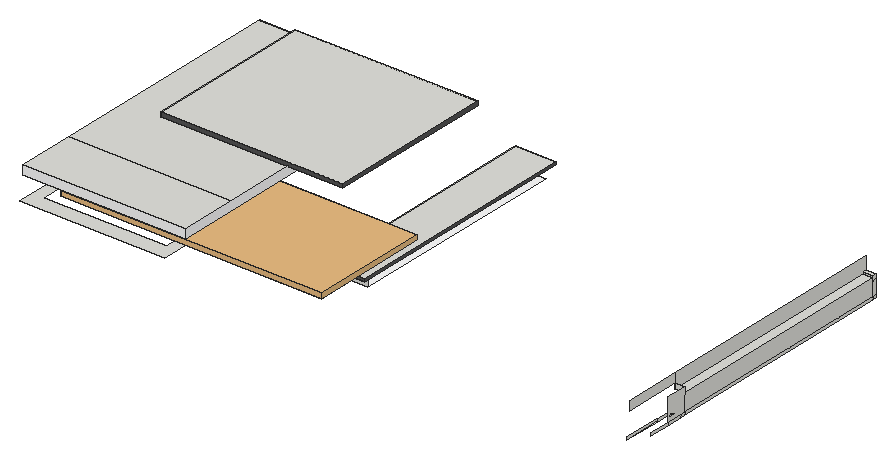
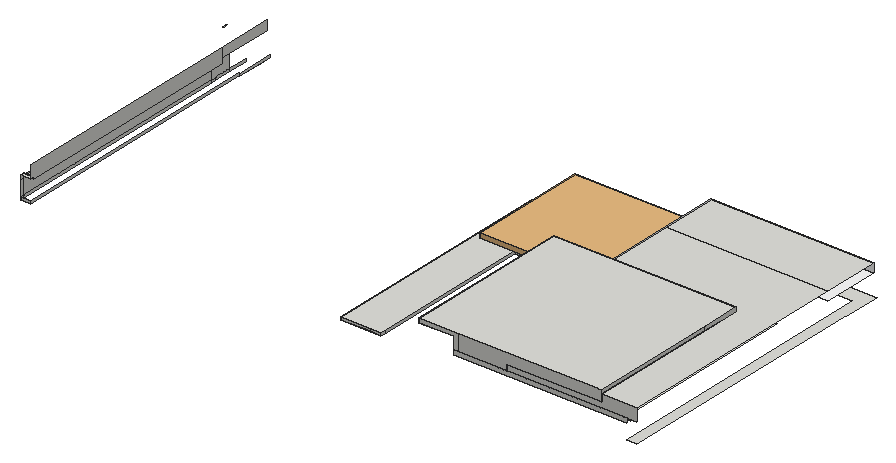
# SketchUp Ruby script. Lengths in inches.
U = 1.inch
M = Sketchup.active_model
def pt(a) = Geom::Point3d.new(a.map { |v| v * U })
def face(e, loops, mat)
  f = e.add_face(loops[0].map { |a| pt(a) })
  loops[1..].each { |l| e.add_face(l.map { |a| pt(a) }).erase! }
  f.material = f.back_material = mat if mat
  f
end
# faces: each face lists its corners as indices into pts; further lists are holes
def faces(e, pts, list, mat = nil) = list.each { |f| face(e, (f[0].is_a?(Array) ? f : [f]).map { |l| l.map { |i| pts[i] } }, mat) }
# xy, xz, yz: faces in a plane at the given z, y or x. An outline is a flat list of corners, or four numbers for a rectangle; further outlines are holes
def ring(l) = l.size == 4 ? [[l[0], l[1]], [l[2], l[1]], [l[2], l[3]], [l[0], l[3]]] : l.each_slice(2).to_a
def flat(e, list, mat, &to3) = list.each { |f| face(e, (f[0].is_a?(Array) ? f : [f]).map { |l| ring(l).map { |u, v| to3.(u, v) } }, mat) }
def xy(e, z, list, mat = nil) = flat(e, list, mat) { |x, y| [x, y, z] }
def xz(e, y, list, mat = nil) = flat(e, list, mat) { |x, z| [x, y, z] }
def yz(e, x, list, mat = nil) = flat(e, list, mat) { |y, z| [x, y, z] }
def lines(e, pts, list) = list.each { |a, b| e.add_line(pt(pts[a]), pt(pts[b])) }
# prism: a flat outline (further loops are holes) pulled along v
def prism(e, loops, v, mat = nil)
  f = face(e, loops, mat); d = Geom::Vector3d.new(v.map { |x| x * U })
  f.pushpull(f.normal.samedirection?(d) ? d.length : -d.length)
end
def box(e, o, s, mat = nil) = prism(e, [[o, [o[0] + s[0], o[1], o[2]], [o[0] + s[0], o[1] + s[1], o[2]], [o[0], o[1] + s[1], o[2]]]], [0, 0, s[2]], mat)
def at(x, y, z, deg = 0) = Geom::Transformation.translation(pt([x, y, z])) * Geom::Transformation.rotation(ORIGIN, Z_AXIS, deg.degrees)
def axes(o, x, y, z) = Geom::Transformation.new([*x, 0, *y, 0, *z, 0, *pt(o).to_a, 1])
def part(name) = M.definitions.add(name)
# library, detail: a bought-in or finely detailed component or shape, given as its bounding box
def library(name, o, s) = part(name).tap { |d| box(d.entities, o, s) }
def detail(e, o, s) = box(e.add_group.entities, o, s)
def put(e, d, t, mat = nil) = e.add_instance(d, t).tap { |i| i.material = mat if mat }
def group(e, t, mat = nil) = e.add_group.tap { |g| g.transformation = t; g.material = mat if mat }.entities
root = M.entities
M.materials.add("[Color M00]").color = [255, 255, 255]
M.materials.add("[Color M06]").color = [86, 86, 86]
c1 = library("Mesh Light\#4",[-0.5,-0.5,-0.1],[1,1,0.2])
c2 = part("Group\#24")
xy(c2.entities,0,[[203.13,95.41,201.58,95.62,200.13,96.22,198.89,97.17,197.9375,98.41,197.34,99.86,197.13,101.41,197.34,102.96,197.9375,104.41,198.89,105.65,200.13,106.61,201.58,107.21,203.13,107.41,204.6875,107.21,206.13,106.61,207.375,105.65,208.33,104.41,208.93,102.96,209.13,101.41,208.93,99.86,208.33,98.41,207.375,97.17,206.13,96.22,204.6875,95.62],[281.57,95.41,280.02,95.62,278.57,96.22,277.33,97.17,276.375,98.41,275.77,99.86,275.57,101.41,275.77,102.96,276.375,104.41,277.33,105.65,278.57,106.61,280.02,107.21,281.57,107.41,283.125,107.21,284.57,106.61,285.8125,105.65,286.77,104.41,287.37,102.96,287.57,101.41,287.37,99.86,286.77,98.41,285.8125,97.17,284.57,96.22,283.125,95.62],[350.95,95.41,349.39,95.62,347.95,96.22,346.7,97.17,345.75,98.41,345.15,99.86,344.95,101.41,345.15,102.96,345.75,104.41,346.7,105.65,347.95,106.61,349.39,107.21,350.95,107.41,352.5,107.21,353.95,106.61,355.1875,105.65,356.14,104.41,356.74,102.96,356.95,101.41,356.74,99.86,356.14,98.41,355.1875,97.17,353.95,96.22,352.5,95.62],[376,162.85,374.44,163.05,373,163.65,371.75,164.6,370.8,165.85,370.2,167.29,370,168.85,370.2,170.4,370.8,171.85,371.75,173.09,373,174.04,374.44,174.64,376,174.85,377.55,174.64,379,174.04,380.24,173.09,381.19,171.85,381.79,170.4,382,168.85,381.79,167.29,381.19,165.85,380.24,164.6,379,163.65,377.55,163.05]],"[Color M00]")
xy(c2.entities,33.4375,[[6,0,4.45,0.2,3,0.8,1.76,1.76,0.8,3,0.2,4.45,0,6,0.2,7.55,0.8,9,1.76,10.24,3,11.2,4.45,11.8,6,12,7.55,11.8,9,11.2,10.24,10.24,11.2,9,11.8,7.55,12,6,11.8,4.45,11.2,3,10.24,1.76,9,0.8,7.55,0.2],[83.125,0,81.57,0.2,80.125,0.8,78.88,1.76,77.93,3,77.33,4.45,77.125,6,77.33,7.55,77.93,9,78.88,10.24,80.125,11.2,81.57,11.8,83.125,12,84.68,11.8,86.125,11.2,87.37,10.24,88.32,9,88.92,7.55,89.125,6,88.92,4.45,88.32,3,87.37,1.76,86.125,0.8,84.68,0.2],[166.6875,0,165.13,0.2,163.6875,0.8,162.44,1.76,161.49,3,160.89,4.45,160.6875,6,160.89,7.55,161.49,9,162.44,10.24,163.6875,11.2,165.13,11.8,166.6875,12,168.24,11.8,169.6875,11.2,170.93,10.24,171.88,9,172.48,7.55,172.6875,6,172.48,4.45,171.88,3,170.93,1.76,169.6875,0.8,168.24,0.2],[166.6875,88.9375,165.13,89.14,163.6875,89.74,162.44,90.69,161.49,91.9375,160.89,93.38,160.6875,94.9375,160.89,96.49,161.49,97.9375,162.44,99.18,163.6875,100.13,165.13,100.73,166.6875,100.9375,168.24,100.73,169.6875,100.13,170.93,99.18,171.88,97.9375,172.48,96.49,172.6875,94.9375,172.48,93.38,171.88,91.9375,170.93,90.69,169.6875,89.74,168.24,89.14]],"[Color M00]")
put(c2.entities,c1,axes([191,87.42,16.72],[382.99758,0,0],[0,175.84579,0],[0,0,34.4375]))
c3 = library("Group\#23",[-0.5,-0.5,-0.1],[13,110.375,0.2])
xy(root,269.375,[[1170.95,1583.41,1383.39,1583.41,1383.39,1676.03,1376.89,1676.03,1376.89,1705.53,1367.875,1705.53,1367.875,1606.6875,1187.0625,1606.6875,1187.0625,2020.66,1172.33,2020.66,1172.33,1638.35,1170.95,1638.35],[1376.89,1676.03,1383.39,1730.6]])
xy(root,269.375,[[[1383.39,1676.03,1383.39,1730.6,1567.08,1730.6,1567.08,2001.02,1607.7,2001.02,1607.7,1676.03],[1418.61,1698.07,1420.16,1698.28,1421.61,1698.875,1422.85,1699.83,1423.8,1701.07,1424.4,1702.52,1424.61,1704.07,1424.4,1705.625,1423.8,1707.07,1422.85,1708.3125,1421.61,1709.27,1420.16,1709.87,1418.61,1710.07,1417.05,1709.87,1415.61,1709.27,1414.36,1708.3125,1413.41,1707.07,1412.81,1705.625,1412.61,1704.07,1412.81,1702.52,1413.41,1701.07,1414.36,1699.83,1415.61,1698.875,1417.05,1698.28],[1497.04,1698.07,1498.6,1698.28,1500.04,1698.875,1501.29,1699.83,1502.24,1701.07,1502.84,1702.52,1503.04,1704.07,1502.84,1705.625,1502.24,1707.07,1501.29,1708.3125,1500.04,1709.27,1498.6,1709.87,1497.04,1710.07,1495.49,1709.87,1494.04,1709.27,1492.8,1708.3125,1491.85,1707.07,1491.25,1705.625,1491.04,1704.07,1491.25,1702.52,1491.85,1701.07,1492.8,1699.83,1494.04,1698.875,1495.49,1698.28],[1566.42,1698.07,1567.97,1698.28,1569.42,1698.875,1570.66,1699.83,1571.61,1701.07,1572.21,1702.52,1572.42,1704.07,1572.21,1705.625,1571.61,1707.07,1570.66,1708.3125,1569.42,1709.27,1567.97,1709.87,1566.42,1710.07,1564.86,1709.87,1563.42,1709.27,1562.17,1708.3125,1561.22,1707.07,1560.62,1705.625,1560.42,1704.07,1560.62,1702.52,1561.22,1701.07,1562.17,1699.83,1563.42,1698.875,1564.86,1698.28],[1591.47,1765.51,1593.02,1765.71,1594.47,1766.31,1595.71,1767.26,1596.67,1768.51,1597.27,1769.95,1597.47,1771.51,1597.27,1773.06,1596.67,1774.51,1595.71,1775.75,1594.47,1776.7,1593.02,1777.3,1591.47,1777.51,1589.92,1777.3,1588.47,1776.7,1587.23,1775.75,1586.27,1774.51,1585.67,1773.06,1585.47,1771.51,1585.67,1769.95,1586.27,1768.51,1587.23,1767.26,1588.47,1766.31,1589.92,1765.71],[1591.47,1845.94,1593.02,1846.15,1594.47,1846.75,1595.71,1847.7,1596.67,1848.94,1597.27,1850.39,1597.47,1851.94,1597.27,1853.5,1596.67,1854.94,1595.71,1856.1875,1594.47,1857.14,1593.02,1857.74,1591.47,1857.94,1589.92,1857.74,1588.47,1857.14,1587.23,1856.1875,1586.27,1854.94,1585.67,1853.5,1585.47,1851.94,1585.67,1850.39,1586.27,1848.94,1587.23,1847.7,1588.47,1846.75,1589.92,1846.15],[1591.47,1943.32,1593.02,1943.52,1594.47,1944.12,1595.71,1945.08,1596.67,1946.32,1597.27,1947.77,1597.47,1949.32,1597.27,1950.87,1596.67,1952.32,1595.71,1953.5625,1594.47,1954.51,1593.02,1955.11,1591.47,1955.32,1589.92,1955.11,1588.47,1954.51,1587.23,1953.5625,1586.27,1952.32,1585.67,1950.87,1585.47,1949.32,1585.67,1947.77,1586.27,1946.32,1587.23,1945.08,1588.47,1944.12,1589.92,1943.52]]],"[Color M00]")
xy(root,270.375,[[2063.54,1592.1,2064.92,1636.04]])
xy(root,279.25,[[1376.89,1669.78,1607.7,1676.03],[1376.89,1676.03,1376.89,1775.97,1548.25,1775.97,1548.25,2020.66,1607.7,2020.66,1607.7,1676.03]])
xy(root,282.6875,[[1376.89,1669.78,1607.7,1669.78,1607.7,2020.66,1548.25,2020.66,1548.25,1775.97,1376.89,1775.97]])
xy(root,291.125,[[1197.375,1733.11,1197.375,2014.29,1364.27,2014.29,1364.27,1853.85,1354.74,1853.85,1354.74,1733.11],[1364.27,1853.85,1434.7,2014.29]])
xy(root,297.875,[[1187.0625,2014.29,1364.27,2020.66],[1364.27,2014.29,1434.7,2020.66]])
xy(root,299.625,[[2064.92,1667.53,2079.65,2011.98]])
xy(root,302.5625,[[2064.92,2011.98,2079.65,2018.36]])
xy(root,302.8125,[[[1172.33,1586.53,1172.33,1669.84,1187.0625,1669.84,1187.0625,1638.53,1364.27,1638.53,1364.27,1831.47,1410.7,1831.47,1410.7,1586.53],[1382.16,1691.6,1383.71,1691.8,1385.16,1692.4,1386.4,1693.35,1387.36,1694.6,1387.96,1696.04,1388.16,1697.6,1387.96,1699.15,1387.36,1700.6,1386.4,1701.84,1385.16,1702.79,1383.71,1703.39,1382.16,1703.6,1380.61,1703.39,1379.16,1702.79,1377.92,1701.84,1376.96,1700.6,1376.36,1699.15,1376.16,1697.6,1376.36,1696.04,1376.96,1694.6,1377.92,1693.35,1379.16,1692.4,1380.61,1691.8],[1221.47,1602.66,1223.03,1602.86,1224.47,1603.46,1225.71,1604.42,1226.67,1605.66,1227.27,1607.11,1227.47,1608.66,1227.27,1610.21,1226.67,1611.66,1225.71,1612.9,1224.47,1613.86,1223.03,1614.46,1221.47,1614.66,1219.92,1614.46,1218.47,1613.86,1217.23,1612.9,1216.28,1611.66,1215.68,1610.21,1215.47,1608.66,1215.68,1607.11,1216.28,1605.66,1217.23,1604.42,1218.47,1603.46,1219.92,1602.86],[1298.6,1602.66,1300.15,1602.86,1301.6,1603.46,1302.84,1604.42,1303.79,1605.66,1304.39,1607.11,1304.6,1608.66,1304.39,1610.21,1303.79,1611.66,1302.84,1612.9,1301.6,1613.86,1300.15,1614.46,1298.6,1614.66,1297.04,1614.46,1295.6,1613.86,1294.35,1612.9,1293.4,1611.66,1292.8,1610.21,1292.6,1608.66,1292.8,1607.11,1293.4,1605.66,1294.35,1604.42,1295.6,1603.46,1297.04,1602.86],[1382.16,1602.66,1383.71,1602.86,1385.16,1603.46,1386.4,1604.42,1387.36,1605.66,1387.96,1607.11,1388.16,1608.66,1387.96,1610.21,1387.36,1611.66,1386.4,1612.9,1385.16,1613.86,1383.71,1614.46,1382.16,1614.66,1380.61,1614.46,1379.16,1613.86,1377.92,1612.9,1376.96,1611.66,1376.36,1610.21,1376.16,1608.66,1376.36,1607.11,1376.96,1605.66,1377.92,1604.42,1379.16,1603.46,1380.61,1602.86]]],"[Color M00]")
xy(root,305.625,[[1224.7,1831.47,1364.27,2020.66]])
xy(root,316.0625,[[1172.33,1586.53,1410.7,1669.84],[1172.33,1669.84,1410.7,1669.84,1410.7,1773.85,1224.7,1773.85,1224.7,2020.66,1172.33,2020.66],[1410.7,1773.85,1410.7,1831.47,1440.7,1831.47,1440.7,2020.66,1492.27,2020.66,1492.27,1773.85]])
xy(root,321.8125,[[1224.7,1773.85,1492.27,2020.66]])
xz(root,1586.53,[[1172.33,302.8125,1410.7,316.0625]],"[Color M00]")
xz(root,1636.04,[[2063.54,270.375,2064.92,274.0625]])
xz(root,1667.53,[[2064.92,299.625,2079.65,307.5]])
xz(root,1669.78,[[1376.89,279.25,1607.7,282.6875]],"[Color M06]")
xz(root,1676.03,[[1376.89,269.375,1607.7,279.25]])
xz(root,1773.85,[[1224.7,316.0625,1492.27,321.8125]],"[Color M06]")
xz(root,1775.97,[[1376.89,279.25,1548.25,282.6875]])
xz(root,1831.47,[[1364.27,302.8125,1410.7,305.625]])
xz(root,2011.98,[[2064.92,299.625,2079.65,302.5625]])
xz(root,2014.29,[[1187.0625,291.125,1364.27,297.875],[1364.27,291.125,1434.7,297.875]])
xz(root,2018.36,[[2064.92,270.375,2079.65,274.0625]])
xz(root,2020.66,[[1548.25,279.25,1563.95,282.6875],[1563.95,279.25,1607.7,282.6875],[1187.0625,291.125,1440.7,297.875],[1172.33,297.875,1172.33,316.0625,1224.7,316.0625,1224.7,305.625,1364.27,305.625,1364.27,297.875],[1364.27,297.875,1364.27,305.625,1224.7,305.625,1224.7,321.8125,1434.7,321.8125,1434.7,297.875],
  [1434.7,297.875,1434.7,321.8125,1492.27,321.8125,1492.27,316.0625,1440.7,316.0625,1440.7,297.875]])
yz(root,1224.7,[[1803.47,305.625,1831.47,316.0625],[1831.47,305.625,2020.66,316.0625],[1773.85,316.0625,1831.47,321.8125],[1831.47,316.0625,2020.66,321.8125]])
yz(root,1364.27,[[1831.47,291.125,2014.29,297.875],[1831.47,297.875,2020.66,305.625]])
yz(root,1376.89,[[1669.78,279.25,1775.97,282.6875]])
yz(root,1410.7,[[1586.53,302.8125,1831.47,316.0625]],"[Color M00]")
yz(root,1492.27,[[1773.85,316.0625,2020.66,321.8125]],"[Color M06]")
yz(root,1548.25,[[1775.97,279.25,2014.29,282.6875],[2014.29,279.25,2020.66,282.6875]])
yz(root,1607.7,[[1669.78,279.25,2020.66,282.6875]],"[Color M06]")
yz(root,2063.54,[[1581.1,270.375,1636.04,274.0625]])
yz(root,2064.92,[[1636.04,270.375,2018.36,274.0625],[1667.53,299.625,1667.53,320.75,2018.36,320.75,2018.36,302.5625,2011.98,302.5625,2011.98,299.625],[1584.22,307.5,1667.53,320.75]])
yz(root,2079.65,[[1604.38,270.375,1636.22,274.0625],[1636.22,270.375,1659.57,274.0625],[1659.57,270.375,1667.53,274.0625],[1667.53,270.375,2011.98,274.0625],[2011.98,270.375,2018.36,274.0625],
  [1636.22,274.0625,1667.53,307.5],[1667.53,274.0625,2011.98,299.625],[2011.98,274.0625,2018.36,295.8125],[2011.98,295.8125,2018.36,302.5625]])
p = [[1418.61,1698.07,269.375],[1417.05,1698.28,269.375],[1417.05,1698.28,270.0625],[1418.61,1698.07,270.0625],[1420.16,1698.28,269.375],[1420.16,1698.28,270.0625],
  [1497.04,1698.07,269.375],[1495.49,1698.28,269.375],[1495.49,1698.28,270.0625],[1497.04,1698.07,270.0625],[1498.6,1698.28,269.375],[1498.6,1698.28,270.0625],
  [1566.42,1698.07,269.375],[1564.86,1698.28,269.375],[1564.86,1698.28,270.0625],[1566.42,1698.07,270.0625],[1567.97,1698.28,269.375],[1567.97,1698.28,270.0625],
  [1415.61,1698.875,269.375],[1415.61,1698.875,270.0625],[1421.61,1698.875,269.375],[1421.61,1698.875,270.0625],[1494.04,1698.875,269.375],[1494.04,1698.875,270.0625],
  [1500.04,1698.875,269.375],[1500.04,1698.875,270.0625],[1563.42,1698.875,269.375],[1563.42,1698.875,270.0625],[1569.42,1698.875,269.375],[1569.42,1698.875,270.0625],
  [1414.36,1699.83,269.375],[1414.36,1699.83,270.0625],[1422.85,1699.83,269.375],[1422.85,1699.83,270.0625],[1492.8,1699.83,269.375],[1492.8,1699.83,270.0625],
  [1501.29,1699.83,269.375],[1501.29,1699.83,270.0625],[1562.17,1699.83,269.375],[1562.17,1699.83,270.0625],[1570.66,1699.83,269.375],[1570.66,1699.83,270.0625],
  [1413.41,1701.07,269.375],[1413.41,1701.07,270.0625],[1423.8,1701.07,269.375],[1423.8,1701.07,270.0625],[1491.85,1701.07,269.375],[1491.85,1701.07,270.0625],
  [1502.24,1701.07,269.375],[1502.24,1701.07,270.0625],[1561.22,1701.07,269.375],[1561.22,1701.07,270.0625],[1571.61,1701.07,269.375],[1571.61,1701.07,270.0625],
  [1412.81,1702.52,269.375],[1412.81,1702.52,270.0625],[1424.4,1702.52,269.375],[1424.4,1702.52,270.0625],[1491.25,1702.52,269.375],[1491.25,1702.52,270.0625],
  [1502.84,1702.52,269.375],[1502.84,1702.52,270.0625],[1560.62,1702.52,269.375],[1560.62,1702.52,270.0625],[1572.21,1702.52,269.375],[1572.21,1702.52,270.0625],
  [1412.61,1704.07,269.375],[1412.61,1704.07,270.0625],[1424.61,1704.07,269.375],[1424.61,1704.07,270.0625],[1491.04,1704.07,269.375],[1491.04,1704.07,270.0625],
  [1503.04,1704.07,269.375],[1503.04,1704.07,270.0625],[1560.42,1704.07,269.375],[1560.42,1704.07,270.0625],[1572.42,1704.07,269.375],[1572.42,1704.07,270.0625],
  [1412.81,1705.625,269.375],[1412.81,1705.625,270.0625],[1424.4,1705.625,269.375],[1424.4,1705.625,270.0625],[1491.25,1705.625,269.375],[1491.25,1705.625,270.0625],
  [1502.84,1705.625,269.375],[1502.84,1705.625,270.0625],[1560.62,1705.625,269.375],[1560.62,1705.625,270.0625],[1572.21,1705.625,269.375],[1572.21,1705.625,270.0625],
  [1413.41,1707.07,269.375],[1413.41,1707.07,270.0625],[1423.8,1707.07,269.375],[1423.8,1707.07,270.0625],[1491.85,1707.07,269.375],[1491.85,1707.07,270.0625],
  [1502.24,1707.07,269.375],[1502.24,1707.07,270.0625],[1561.22,1707.07,269.375],[1561.22,1707.07,270.0625],[1571.61,1707.07,269.375],[1571.61,1707.07,270.0625],
  [1414.36,1708.3125,269.375],[1414.36,1708.3125,270.0625],[1422.85,1708.3125,269.375],[1422.85,1708.3125,270.0625],[1492.8,1708.3125,269.375],[1492.8,1708.3125,270.0625],
  [1501.29,1708.3125,269.375],[1501.29,1708.3125,270.0625],[1562.17,1708.3125,269.375],[1562.17,1708.3125,270.0625],[1570.66,1708.3125,269.375],[1570.66,1708.3125,270.0625],
  [1415.61,1709.27,269.375],[1415.61,1709.27,270.0625],[1421.61,1709.27,269.375],[1421.61,1709.27,270.0625],[1494.04,1709.27,269.375],[1494.04,1709.27,270.0625],
  [1500.04,1709.27,269.375],[1500.04,1709.27,270.0625],[1563.42,1709.27,269.375],[1563.42,1709.27,270.0625],[1569.42,1709.27,269.375],[1569.42,1709.27,270.0625],
  [1417.05,1709.87,269.375],[1417.05,1709.87,270.0625],[1420.16,1709.87,269.375],[1420.16,1709.87,270.0625],[1495.49,1709.87,269.375],[1495.49,1709.87,270.0625],
  [1498.6,1709.87,269.375],[1498.6,1709.87,270.0625],[1564.86,1709.87,269.375],[1564.86,1709.87,270.0625],[1567.97,1709.87,269.375],[1567.97,1709.87,270.0625],
  [1418.61,1710.07,269.375],[1418.61,1710.07,270.0625],[1497.04,1710.07,269.375],[1497.04,1710.07,270.0625],[1566.42,1710.07,269.375],[1566.42,1710.07,270.0625],
  [1591.47,1765.51,269.375],[1589.92,1765.71,269.375],[1589.92,1765.71,270.0625],[1591.47,1765.51,270.0625],[1593.02,1765.71,269.375],[1593.02,1765.71,270.0625],
  [1588.47,1766.31,269.375],[1588.47,1766.31,270.0625],[1594.47,1766.31,269.375],[1594.47,1766.31,270.0625],[1587.23,1767.26,269.375],[1587.23,1767.26,270.0625],
  [1595.71,1767.26,269.375],[1595.71,1767.26,270.0625],[1586.27,1768.51,269.375],[1586.27,1768.51,270.0625],[1596.67,1768.51,269.375],[1596.67,1768.51,270.0625],
  [1585.67,1769.95,269.375],[1585.67,1769.95,270.0625],[1597.27,1769.95,269.375],[1597.27,1769.95,270.0625],[1585.47,1771.51,269.375],[1585.47,1771.51,270.0625],
  [1597.47,1771.51,269.375],[1597.47,1771.51,270.0625],[1585.67,1773.06,269.375],[1585.67,1773.06,270.0625],[1597.27,1773.06,269.375],[1597.27,1773.06,270.0625],
  [1586.27,1774.51,269.375],[1586.27,1774.51,270.0625],[1596.67,1774.51,269.375],[1596.67,1774.51,270.0625],[1587.23,1775.75,269.375],[1587.23,1775.75,270.0625],
  [1595.71,1775.75,269.375],[1595.71,1775.75,270.0625],[1588.47,1776.7,269.375],[1588.47,1776.7,270.0625],[1594.47,1776.7,269.375],[1594.47,1776.7,270.0625],
  [1589.92,1777.3,269.375],[1589.92,1777.3,270.0625],[1593.02,1777.3,269.375],[1593.02,1777.3,270.0625],[1591.47,1777.51,269.375],[1591.47,1777.51,270.0625],
  [1591.47,1845.94,269.375],[1589.92,1846.15,269.375],[1589.92,1846.15,270.0625],[1591.47,1845.94,270.0625],[1593.02,1846.15,269.375],[1593.02,1846.15,270.0625],
  [1588.47,1846.75,269.375],[1588.47,1846.75,270.0625],[1594.47,1846.75,269.375],[1594.47,1846.75,270.0625],[1587.23,1847.7,269.375],[1587.23,1847.7,270.0625],
  [1595.71,1847.7,269.375],[1595.71,1847.7,270.0625],[1586.27,1848.94,269.375],[1586.27,1848.94,270.0625],[1596.67,1848.94,269.375],[1596.67,1848.94,270.0625],
  [1585.67,1850.39,269.375],[1585.67,1850.39,270.0625],[1597.27,1850.39,269.375],[1597.27,1850.39,270.0625],[1585.47,1851.94,269.375],[1585.47,1851.94,270.0625],
  [1597.47,1851.94,269.375],[1597.47,1851.94,270.0625],[1585.67,1853.5,269.375],[1585.67,1853.5,270.0625],[1597.27,1853.5,269.375],[1597.27,1853.5,270.0625],
  [1586.27,1854.94,269.375],[1586.27,1854.94,270.0625],[1596.67,1854.94,269.375],[1596.67,1854.94,270.0625],[1587.23,1856.1875,269.375],[1587.23,1856.1875,270.0625],
  [1595.71,1856.1875,269.375],[1595.71,1856.1875,270.0625],[1588.47,1857.14,269.375],[1588.47,1857.14,270.0625],[1594.47,1857.14,269.375],[1594.47,1857.14,270.0625],
  [1589.92,1857.74,269.375],[1589.92,1857.74,270.0625],[1593.02,1857.74,269.375],[1593.02,1857.74,270.0625],[1591.47,1857.94,269.375],[1591.47,1857.94,270.0625],
  [1591.47,1943.32,269.375],[1589.92,1943.52,269.375],[1589.92,1943.52,270.0625],[1591.47,1943.32,270.0625],[1593.02,1943.52,269.375],[1593.02,1943.52,270.0625],
  [1588.47,1944.12,269.375],[1588.47,1944.12,270.0625],[1594.47,1944.12,269.375],[1594.47,1944.12,270.0625],[1587.23,1945.08,269.375],[1587.23,1945.08,270.0625],
  [1595.71,1945.08,269.375],[1595.71,1945.08,270.0625],[1586.27,1946.32,269.375],[1586.27,1946.32,270.0625],[1596.67,1946.32,269.375],[1596.67,1946.32,270.0625],
  [1585.67,1947.77,269.375],[1585.67,1947.77,270.0625],[1597.27,1947.77,269.375],[1597.27,1947.77,270.0625],[1585.47,1949.32,269.375],[1585.47,1949.32,270.0625],
  [1597.47,1949.32,269.375],[1597.47,1949.32,270.0625],[1585.67,1950.87,269.375],[1585.67,1950.87,270.0625],[1597.27,1950.87,269.375],[1597.27,1950.87,270.0625],
  [1586.27,1952.32,269.375],[1586.27,1952.32,270.0625],[1596.67,1952.32,269.375],[1596.67,1952.32,270.0625],[1587.23,1953.5625,269.375],[1587.23,1953.5625,270.0625],
  [1595.71,1953.5625,269.375],[1595.71,1953.5625,270.0625],[1588.47,1954.51,269.375],[1588.47,1954.51,270.0625],[1594.47,1954.51,269.375],[1594.47,1954.51,270.0625],
  [1589.92,1955.11,269.375],[1589.92,1955.11,270.0625],[1593.02,1955.11,269.375],[1593.02,1955.11,270.0625],[1591.47,1955.32,269.375],[1591.47,1955.32,270.0625],
  [1221.47,1602.66,302.8125],[1219.92,1602.86,302.8125],[1219.92,1602.86,303.5],[1221.47,1602.66,303.5],[1223.03,1602.86,302.8125],[1223.03,1602.86,303.5],
  [1298.6,1602.66,302.8125],[1297.04,1602.86,302.8125],[1297.04,1602.86,303.5],[1298.6,1602.66,303.5],[1300.15,1602.86,302.8125],[1300.15,1602.86,303.5],
  [1382.16,1602.66,302.8125],[1380.61,1602.86,302.8125],[1380.61,1602.86,303.5],[1382.16,1602.66,303.5],[1383.71,1602.86,302.8125],[1383.71,1602.86,303.5],
  [1218.47,1603.46,302.8125],[1218.47,1603.46,303.5],[1224.47,1603.46,302.8125],[1224.47,1603.46,303.5],[1295.6,1603.46,302.8125],[1295.6,1603.46,303.5],
  [1301.6,1603.46,302.8125],[1301.6,1603.46,303.5],[1379.16,1603.46,302.8125],[1379.16,1603.46,303.5],[1385.16,1603.46,302.8125],[1385.16,1603.46,303.5],
  [1217.23,1604.42,302.8125],[1217.23,1604.42,303.5],[1225.71,1604.42,302.8125],[1225.71,1604.42,303.5],[1294.35,1604.42,302.8125],[1294.35,1604.42,303.5],
  [1302.84,1604.42,302.8125],[1302.84,1604.42,303.5],[1377.92,1604.42,302.8125],[1377.92,1604.42,303.5],[1386.4,1604.42,302.8125],[1386.4,1604.42,303.5],
  [1216.28,1605.66,302.8125],[1216.28,1605.66,303.5],[1226.67,1605.66,302.8125],[1226.67,1605.66,303.5],[1293.4,1605.66,302.8125],[1293.4,1605.66,303.5],
  [1303.79,1605.66,302.8125],[1303.79,1605.66,303.5],[1376.96,1605.66,302.8125],[1376.96,1605.66,303.5],[1387.36,1605.66,302.8125],[1387.36,1605.66,303.5],
  [1215.68,1607.11,302.8125],[1215.68,1607.11,303.5],[1227.27,1607.11,302.8125],[1227.27,1607.11,303.5],[1292.8,1607.11,302.8125],[1292.8,1607.11,303.5],
  [1304.39,1607.11,302.8125],[1304.39,1607.11,303.5],[1376.36,1607.11,302.8125],[1376.36,1607.11,303.5],[1387.96,1607.11,302.8125],[1387.96,1607.11,303.5],
  [1227.47,1608.66,302.8125],[1227.47,1608.66,303.5],[1292.6,1608.66,302.8125],[1292.6,1608.66,303.5],[1304.6,1608.66,302.8125],[1304.6,1608.66,303.5],
  [1376.16,1608.66,302.8125],[1376.16,1608.66,303.5],[1388.16,1608.66,302.8125],[1388.16,1608.66,303.5],[1227.27,1610.21,302.8125],[1227.27,1610.21,303.5],
  [1292.8,1610.21,302.8125],[1292.8,1610.21,303.5],[1304.39,1610.21,302.8125],[1304.39,1610.21,303.5],[1376.36,1610.21,302.8125],[1376.36,1610.21,303.5],
  [1387.96,1610.21,302.8125],[1387.96,1610.21,303.5],[1215.68,1610.21,302.8125],[1216.28,1611.66,302.8125],[1216.28,1611.66,303.5],[1215.68,1610.21,303.5],
  [1226.67,1611.66,302.8125],[1226.67,1611.66,303.5],[1293.4,1611.66,302.8125],[1293.4,1611.66,303.5],[1303.79,1611.66,302.8125],[1303.79,1611.66,303.5],
  [1376.96,1611.66,302.8125],[1376.96,1611.66,303.5],[1387.36,1611.66,302.8125],[1387.36,1611.66,303.5],[1217.23,1612.9,302.8125],[1217.23,1612.9,303.5],
  [1225.71,1612.9,302.8125],[1225.71,1612.9,303.5],[1294.35,1612.9,302.8125],[1294.35,1612.9,303.5],[1302.84,1612.9,302.8125],[1302.84,1612.9,303.5],
  [1377.92,1612.9,302.8125],[1377.92,1612.9,303.5],[1386.4,1612.9,302.8125],[1386.4,1612.9,303.5],[1218.47,1613.86,302.8125],[1218.47,1613.86,303.5],
  [1224.47,1613.86,302.8125],[1224.47,1613.86,303.5],[1295.6,1613.86,302.8125],[1295.6,1613.86,303.5],[1301.6,1613.86,302.8125],[1301.6,1613.86,303.5],
  [1379.16,1613.86,302.8125],[1379.16,1613.86,303.5],[1385.16,1613.86,302.8125],[1385.16,1613.86,303.5],[1219.92,1614.46,302.8125],[1219.92,1614.46,303.5],
  [1223.03,1614.46,302.8125],[1223.03,1614.46,303.5],[1297.04,1614.46,302.8125],[1297.04,1614.46,303.5],[1300.15,1614.46,302.8125],[1300.15,1614.46,303.5],
  [1380.61,1614.46,302.8125],[1380.61,1614.46,303.5],[1383.71,1614.46,302.8125],[1383.71,1614.46,303.5],[1221.47,1614.66,302.8125],[1221.47,1614.66,303.5],
  [1298.6,1614.66,302.8125],[1298.6,1614.66,303.5],[1382.16,1614.66,302.8125],[1382.16,1614.66,303.5],[1382.16,1691.6,302.8125],[1380.61,1691.8,302.8125],
  [1380.61,1691.8,303.5],[1382.16,1691.6,303.5],[1383.71,1691.8,302.8125],[1383.71,1691.8,303.5],[1379.16,1692.4,302.8125],[1379.16,1692.4,303.5],
  [1385.16,1692.4,302.8125],[1385.16,1692.4,303.5],[1377.92,1693.35,302.8125],[1377.92,1693.35,303.5],[1386.4,1693.35,302.8125],[1386.4,1693.35,303.5],
  [1376.96,1694.6,302.8125],[1376.96,1694.6,303.5],[1387.36,1694.6,302.8125],[1387.36,1694.6,303.5],[1376.36,1696.04,302.8125],[1376.36,1696.04,303.5],
  [1387.96,1696.04,302.8125],[1387.96,1696.04,303.5],[1376.16,1697.6,302.8125],[1376.16,1697.6,303.5],[1388.16,1697.6,302.8125],[1388.16,1697.6,303.5],
  [1376.36,1699.15,302.8125],[1376.36,1699.15,303.5],[1387.96,1699.15,302.8125],[1387.96,1699.15,303.5],[1376.96,1700.6,302.8125],[1376.96,1700.6,303.5],
  [1387.36,1700.6,302.8125],[1387.36,1700.6,303.5],[1377.92,1701.84,302.8125],[1377.92,1701.84,303.5],[1386.4,1701.84,302.8125],[1386.4,1701.84,303.5],
  [1379.16,1702.79,302.8125],[1379.16,1702.79,303.5],[1385.16,1702.79,302.8125],[1385.16,1702.79,303.5],[1380.61,1703.39,302.8125],[1380.61,1703.39,303.5],
  [1383.71,1703.39,302.8125],[1383.71,1703.39,303.5],[1382.16,1703.6,302.8125],[1382.16,1703.6,303.5],[2108.87,1603.35,307.5],[2108.27,1604.8,307.5],
  [2108.27,1604.8,308.1875],[2108.87,1603.35,308.1875],[2108.0625,1606.35,307.5],[2108.0625,1606.35,308.1875],[2108.27,1607.91,307.5],[2108.27,1607.91,308.1875],
  [2108.87,1609.35,307.5],[2108.87,1609.35,308.1875],[2089.96,1730.8,295.8125],[2079.65,1730.8,295.8125],[1434.7,2014.29,297.875],[1434.7,1831.47,297.875],
  [1434.7,1853.85,291.125],[1440.7,1853.85,291.125],[1567.08,2001.02,269.375],[1567.08,2001.02,277.5],[1434.7,1831.47,291.125],[1224.7,1803.47,305.625],
  [1394.33,1803.47,305.625]]
faces(root,p,[[0,1,2,3],[4,0,3,5],[6,7,8,9],[10,6,9,11],[12,13,14,15],[16,12,15,17],[1,18,19,2],[20,4,5,21],
  [7,22,23,8],[24,10,11,25],[13,26,27,14],[28,16,17,29],[18,30,31,19],[32,20,21,33],[22,34,35,23],[36,24,25,37],
  [26,38,39,27],[40,28,29,41],[30,42,43,31],[44,32,33,45],[34,46,47,35],[48,36,37,49],[38,50,51,39],[52,40,41,53],
  [42,54,55,43],[56,44,45,57],[46,58,59,47],[60,48,49,61],[50,62,63,51],[64,52,53,65],[54,66,67,55],[68,56,57,69],
  [58,70,71,59],[72,60,61,73],[62,74,75,63],[76,64,65,77],[66,78,79,67],[80,68,69,81],[70,82,83,71],[84,72,73,85],
  [74,86,87,75],[88,76,77,89],[78,90,91,79],[92,80,81,93],[82,94,95,83],[96,84,85,97],[86,98,99,87],[100,88,89,101],
  [90,102,103,91],[104,92,93,105],[94,106,107,95],[108,96,97,109],[98,110,111,99],[112,100,101,113],[102,114,115,103],[116,104,105,117],
  [106,118,119,107],[120,108,109,121],[110,122,123,111],[124,112,113,125],[114,126,127,115],[128,116,117,129],[118,130,131,119],[132,120,121,133],
  [122,134,135,123],[136,124,125,137],[126,138,139,127],[138,128,129,139],[130,140,141,131],[140,132,133,141],[134,142,143,135],[142,136,137,143],
  [144,145,146,147],[148,144,147,149],[145,150,151,146],[152,148,149,153],[150,154,155,151],[156,152,153,157],[154,158,159,155],[160,156,157,161],
  [158,162,163,159],[164,160,161,165],[162,166,167,163],[168,164,165,169],[166,170,171,167],[172,168,169,173],[170,174,175,171],[176,172,173,177],
  [174,178,179,175],[180,176,177,181],[178,182,183,179],[184,180,181,185],[182,186,187,183],[188,184,185,189],[186,190,191,187],[190,188,189,191],
  [192,193,194,195],[196,192,195,197],[193,198,199,194],[200,196,197,201],[198,202,203,199],[204,200,201,205],[202,206,207,203],[208,204,205,209],
  [206,210,211,207],[212,208,209,213],[210,214,215,211],[216,212,213,217],[214,218,219,215],[220,216,217,221],[218,222,223,219],[224,220,221,225],
  [222,226,227,223],[228,224,225,229],[226,230,231,227],[232,228,229,233],[230,234,235,231],[236,232,233,237],[234,238,239,235],[238,236,237,239],
  [240,241,242,243],[244,240,243,245],[241,246,247,242],[248,244,245,249],[246,250,251,247],[252,248,249,253],[250,254,255,251],[256,252,253,257],
  [254,258,259,255],[260,256,257,261],[258,262,263,259],[264,260,261,265],[262,266,267,263],[268,264,265,269],[266,270,271,267],[272,268,269,273],
  [270,274,275,271],[276,272,273,277],[274,278,279,275],[280,276,277,281],[278,282,283,279],[284,280,281,285],[282,286,287,283],[286,284,285,287],
  [288,289,290,291],[292,288,291,293],[294,295,296,297],[298,294,297,299],[300,301,302,303],[304,300,303,305],[289,306,307,290],[308,292,293,309],
  [295,310,311,296],[312,298,299,313],[301,314,315,302],[316,304,305,317],[306,318,319,307],[320,308,309,321],[310,322,323,311],[324,312,313,325],
  [314,326,327,315],[328,316,317,329],[318,330,331,319],[332,320,321,333],[322,334,335,323],[336,324,325,337],[326,338,339,327],[340,328,329,341],
  [330,342,343,331],[344,332,333,345],[334,346,347,335],[348,336,337,349],[338,350,351,339],[352,340,341,353],[354,344,345,355],[346,356,357,347],
  [358,348,349,359],[350,360,361,351],[362,352,353,363],[364,354,355,365],[356,366,367,357],[368,358,359,369],[360,370,371,361],[372,362,363,373],
  [374,375,376,377],[378,364,365,379],[366,380,381,367],[382,368,369,383],[370,384,385,371],[386,372,373,387],[375,388,389,376],[390,378,379,391],
  [380,392,393,381],[394,382,383,395],[384,396,397,385],[398,386,387,399],[388,400,401,389],[402,390,391,403],[392,404,405,393],[406,394,395,407],
  [396,408,409,397],[410,398,399,411],[400,412,413,401],[414,402,403,415],[404,416,417,405],[418,406,407,419],[408,420,421,409],[422,410,411,423],
  [412,424,425,413],[424,414,415,425],[416,426,427,417],[426,418,419,427],[420,428,429,421],[428,422,423,429],[430,431,432,433],[434,430,433,435],
  [431,436,437,432],[438,434,435,439],[436,440,441,437],[442,438,439,443],[440,444,445,441],[446,442,443,447],[444,448,449,445],[450,446,447,451],
  [448,452,453,449],[454,450,451,455],[452,456,457,453],[458,454,455,459],[456,460,461,457],[462,458,459,463],[460,464,465,461],[466,462,463,467],
  [464,468,469,465],[470,466,467,471],[468,472,473,469],[474,470,471,475],[472,476,477,473],[476,474,475,477],[478,479,480,481],[479,482,483,480],
  [482,484,485,483],[484,486,487,485]],"[Color M00]")
lines(root,p,[[488,489],[490,491],[492,493],[494,495],[492,496],[497,498]])
put(root,c2,at(1215.47,1602.66,270.0625))
put(root,c3,at(1585.47,1845.94,270.0625))
